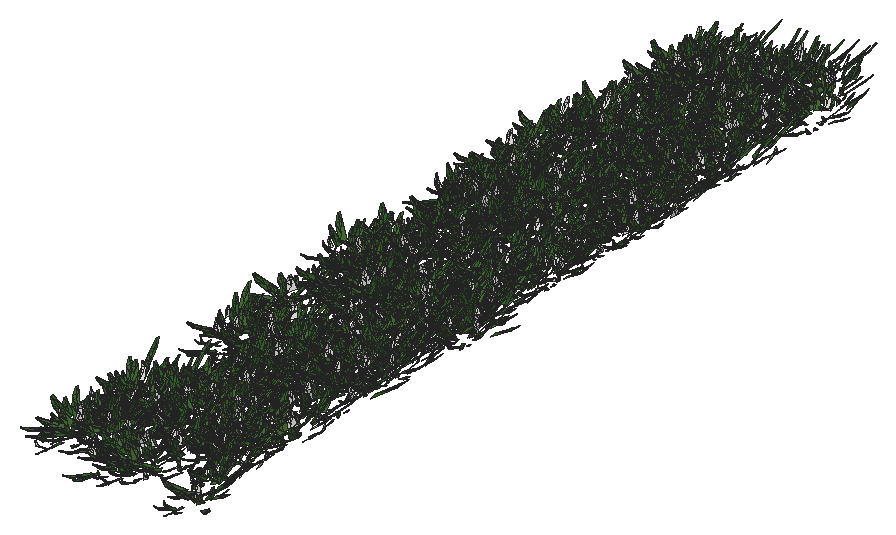
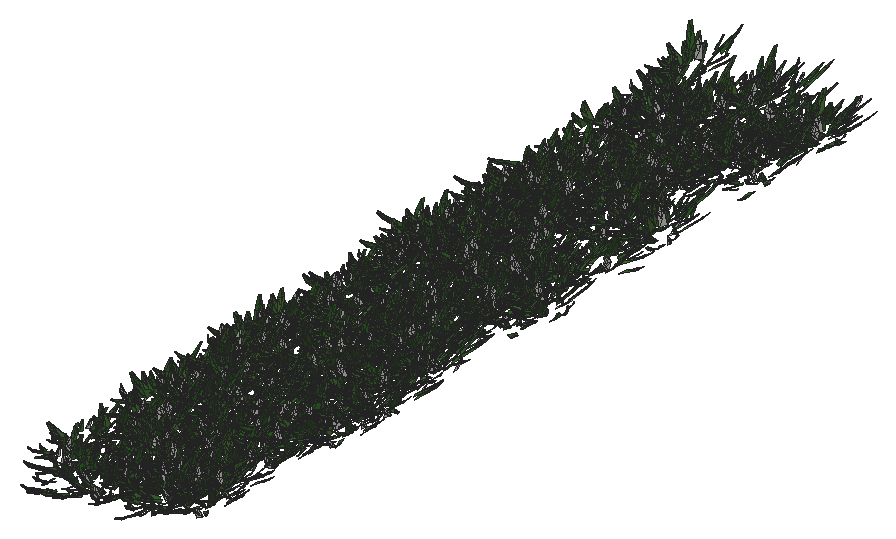
# SketchUp Ruby script. Lengths in inches.
U = 1.inch
M = Sketchup.active_model
def pt(a) = Geom::Point3d.new(a.map { |v| v * U })
def face(e, loops, mat)
  f = e.add_face(loops[0].map { |a| pt(a) })
  loops[1..].each { |l| e.add_face(l.map { |a| pt(a) }).erase! }
  f.material = f.back_material = mat if mat
  f
end
# faces: each face lists its corners as indices into pts; further lists are holes
def faces(e, pts, list, mat = nil) = list.each { |f| face(e, (f[0].is_a?(Array) ? f : [f]).map { |l| l.map { |i| pts[i] } }, mat) }
# xy, xz, yz: faces in a plane at the given z, y or x. An outline is a flat list of corners, or four numbers for a rectangle; further outlines are holes
def ring(l) = l.size == 4 ? [[l[0], l[1]], [l[2], l[1]], [l[2], l[3]], [l[0], l[3]]] : l.each_slice(2).to_a
def flat(e, list, mat, &to3) = list.each { |f| face(e, (f[0].is_a?(Array) ? f : [f]).map { |l| ring(l).map { |u, v| to3.(u, v) } }, mat) }
def xy(e, z, list, mat = nil) = flat(e, list, mat) { |x, y| [x, y, z] }
def xz(e, y, list, mat = nil) = flat(e, list, mat) { |x, z| [x, y, z] }
def yz(e, x, list, mat = nil) = flat(e, list, mat) { |y, z| [x, y, z] }
def lines(e, pts, list) = list.each { |a, b| e.add_line(pt(pts[a]), pt(pts[b])) }
# prism: a flat outline (further loops are holes) pulled along v
def prism(e, loops, v, mat = nil)
  f = face(e, loops, mat); d = Geom::Vector3d.new(v.map { |x| x * U })
  f.pushpull(f.normal.samedirection?(d) ? d.length : -d.length)
end
def box(e, o, s, mat = nil) = prism(e, [[o, [o[0] + s[0], o[1], o[2]], [o[0] + s[0], o[1] + s[1], o[2]], [o[0], o[1] + s[1], o[2]]]], [0, 0, s[2]], mat)
def at(x, y, z, deg = 0) = Geom::Transformation.translation(pt([x, y, z])) * Geom::Transformation.rotation(ORIGIN, Z_AXIS, deg.degrees)
def axes(o, x, y, z) = Geom::Transformation.new([*x, 0, *y, 0, *z, 0, *pt(o).to_a, 1])
def part(name) = M.definitions.add(name)
# library, detail: a bought-in or finely detailed component or shape, given as its bounding box
def library(name, o, s) = part(name).tap { |d| box(d.entities, o, s) }
def detail(e, o, s) = box(e.add_group.entities, o, s)
def put(e, d, t, mat = nil) = e.add_instance(d, t).tap { |i| i.material = mat if mat }
def group(e, t, mat = nil) = e.add_group.tap { |g| g.transformation = t; g.material = mat if mat }.entities
root = M.entities
M.materials.add("Material10").color = [48, 90, 38]
M.materials.add("Material11").color = [68, 110, 48]
M.materials.add("Material12").color = [48, 90, 48]
M.materials.add("Material13").color = [58, 110, 58]
M.materials.add("Material14").color = [58, 90, 38]
M.materials.add("Material15").color = [68, 100, 58]
M.materials.add("Material16").color = [48, 100, 38]
M.materials.add("Material9").color = [68, 110, 58]
c1 = part("grass00")
p = [[-0.6875,0.15,0],[-0.56,0.08,5.52],[-0.04,0.03,2.76],[0.48,-0.02,0],[0.35,-0.02,5.52],[-0.1,-0.14,5.52],
  [-0.12,0.65,8.37],[-0.42,0.65,8.37]]
faces(c1.entities,p,[[0,1,2,3],[3,2,4],[1,5,2],[5,4,2],[1,6,5],[4,5,6],[7,6,1]])
c2 = part("Group16\#1")
put(c2.entities,c1,axes([1.44,-0.61,-0.01],[0.05352,0.12609,0],[-0.10704,0.04543,0.07239],[0.06664,-0.02828,0.11628]),"Material12")
put(c2.entities,c1,axes([0.76,-0.15,-0.01],[0.04676,0.24062,0],[-0.23162,0.04501,0.06642],[0.0652,-0.01267,0.23595]),"Material9")
put(c2.entities,c1,axes([0.79,0.01,-0.01],[-0.00606,0.34651,0],[-0.34381,-0.00602,0.0432],[0.04319,0.00076,0.34386]))
put(c2.entities,c1,axes([1,0.23,-0.01],[-0.07192,0.31144,0],[-0.28722,-0.06632,0.1236],[0.12043,0.02781,0.29478]),"Material11")
put(c2.entities,c1,axes([1.66,0.77,-0.01],[-0.13828,0.29651,0],[-0.21551,-0.1005,0.22471],[0.20365,0.09498,0.23779]),"Material16")
put(c2.entities,c1,axes([0.6875,0.52,-0.01],[-0.18126,0.24051,0],[-0.22746,-0.17142,0.09788],[0.07817,0.05891,0.28481]),"Material11")
put(c2.entities,c1,axes([0.68,0.78,-0.01],[-0.215,0.18688,0],[-0.12385,-0.14248,0.21334],[0.13995,0.16101,0.18878]),"Material9")
put(c2.entities,c1,axes([0.56,1,-0.01],[-0.13756,0.07624,0],[-0.06159,-0.11112,0.0927],[0.04494,0.08108,0.12705]),"Material11")
put(c2.entities,c1,axes([0.2,0.64,-0.01],[-0.23729,0.07254,0],[-0.05711,-0.18681,0.153],[0.04473,0.14632,0.19535]),"Material16")
put(c2.entities,c1,axes([0.0625,0.72,-0.01],[-0.28874,0.02525,0],[-0.02179,-0.24916,0.14647],[0.01276,0.14591,0.25012]),"Material9")
put(c2.entities,c1,axes([-0.08,0.62,-0.01],[-0.34089,-0.04187,0],[0.03255,-0.26504,0.216],[-0.02633,0.21439,0.26703]),"Material16")
put(c2.entities,c1,axes([-0.34,0.98,-0.01],[-0.14314,-0.0493,0],[0.04397,-0.12769,0.06843],[-0.02228,0.0647,0.13505]),"Material16")
put(c2.entities,c1,axes([-0.87,1.45,-0.01],[-0.23488,-0.14114,0],[0.13761,-0.22901,0.06087],[-0.03135,0.05217,0.26717]))
put(c2.entities,c1,axes([-0.72,0.77,-0.01],[-0.14208,-0.13251,0],[0.07209,-0.0773,0.16301],[-0.11118,0.11922,0.1057]),"Material16")
put(c2.entities,c1,axes([-0.62,0.43,-0.01],[-0.14845,-0.21203,0],[0.18654,-0.13061,0.12304],[-0.10079,0.07057,0.22772]),"Material9")
put(c2.entities,c1,axes([-0.68,0.29,-0.01],[-0.13639,-0.32136,0],[0.31723,-0.13464,0.05579],[-0.05136,0.0218,0.34462]),"Material10")
put(c2.entities,c1,axes([-0.64,0.125,-0.01],[-0.0458,-0.23569,0],[0.22124,-0.043,0.08276],[-0.08124,0.01579,0.22538]),"Material13")
put(c2.entities,c1,axes([-1.6,-0.03,-0.01],[0.00576,-0.32897,0],[0.27526,0.00482,0.18018],[-0.18015,-0.00315,0.2753]),"Material11")
put(c2.entities,c1,axes([-1.36,-0.31,-0.01],[0.05718,-0.24765,0],[0.18172,0.04196,0.17267],[-0.16825,-0.03885,0.1865]),"Material16")
put(c2.entities,c1,axes([-1.54,-0.72,-0.01],[0.06537,-0.14017,0],[0.13555,0.06321,0.03939],[-0.0357,-0.01665,0.14956]))
put(c2.entities,c1,axes([-1.19,-0.9,-0.01],[0.09597,-0.12735,0],[0.11214,0.08451,0.07557],[-0.06035,-0.04548,0.14042]),"Material15")
put(c2.entities,c1,axes([-0.47,-0.54,-0.01],[0.11588,-0.10072,0],[0.0618,0.0711,0.12124],[-0.07953,-0.0915,0.0942]))
put(c2.entities,c1,axes([-0.47,-0.84,-0.01],[0.11927,-0.0661,0],[0.06603,0.11913,0.00646],[-0.00313,-0.00565,0.13621]),"Material11")
put(c2.entities,c1,axes([-0.38,-1.24,-0.01],[0.28037,-0.08571,0],[0.0618,0.20215,0.20315],[-0.05939,-0.19428,0.21139]),"Material15")
put(c2.entities,c1,axes([-0.06,-0.66,-0.01],[0.22719,-0.01987,0],[0.01247,0.14255,0.17758],[-0.01547,-0.17691,0.1431]),"Material14")
put(c2.entities,c1,axes([0.11,-0.89,-0.01],[0.14882,0.01828,0],[-0.01058,0.08611,0.12229],[0.01491,-0.12138,0.08676]),"Material12")
put(c2.entities,c1,axes([0.25,-0.72,-0.01],[0.20481,0.07053,0],[-0.06206,0.18022,0.10291],[0.03351,-0.0973,0.1906]),"Material12")
put(c2.entities,c1,axes([0.85,-1.42,-0.01],[0.16481,0.09904,0],[-0.09472,0.15762,0.05616],[0.02893,-0.04814,0.18389]),"Material11")
put(c2.entities,c1,axes([1.01,-1.09,-0.01],[0.21858,0.20385,0],[-0.17495,0.1876,0.15339],[0.10462,-0.11218,0.25652]),"Material16")
put(c2.entities,c1,axes([1.01,-0.71,-0.01],[0.08733,0.12473,0],[-0.06445,0.04512,0.13037],[0.1068,-0.07477,0.07867]),"Material12")
c3 = part("Group15\#1")
put(c3.entities,c2,at(0,0,0))
c4 = part("3darcstudiotree_grass00\#1")
put(c4.entities,c3,at(0,0,0))
put(root,c4,axes([935.18,263.3,12.99],[2.16357,-5.91356,0],[2.30527,4.40706,-0.02296],[0.07841,0.1499,1.8355]))
put(root,c4,axes([915.44,263.39,12.99],[-2.20379,4.7227,0],[-1.94764,-4.7489,-0.04557],[-0.15642,-0.38139,1.96028]))
put(root,c4,axes([909.77,264.4,12.99],[0.55955,7.10793,0],[-3.43066,1.41116,-0.03105],[-0.09608,0.03952,1.50318]))
put(root,c4,axes([890.625,270.69,12.99],[2.4509,-2.72765,0],[1.3443,6.31156,-0.02466],[0.03839,0.18026,1.49812]))
put(root,c4,axes([902.12,270.59,12.99],[3.0266,0.5357,0],[-0.23389,6.90474,-0.0417],[-0.01483,0.43784,1.91485]))
put(root,c4,axes([893.11,269.13,12.99],[-2.69886,4.09648,0],[-1.88583,-6.49197,-0.05111],[-0.09296,-0.32002,1.53759]))
put(root,c4,axes([913.71,270.64,12.99],[-2.55155,1.15726,0],[-0.67109,-7.73133,-0.05548],[-0.03755,-0.43264,1.6451]))
put(root,c4,axes([896.61,273.32,12.99],[2.47649,-1.87564,0],[0.81946,5.65356,-0.03222],[0.0507,0.34977,1.78787]))
put(root,c4,axes([933.94,274.82,12.99],[0.26058,-5.98951,0],[2.59588,0.59011,-0.03727],[0.17952,0.04081,1.73202]))
put(root,c4,axes([922.55,274.69,12.99],[2.18042,5.99333,0],[-2.41636,4.59344,-0.02991],[-0.10428,0.19824,1.95467]))
put(root,c4,axes([915.3,280.95,12.99],[0.84248,-6.06099,0],[3.32927,2.41806,-0.03698],[0.1346,0.09776,1.82987]))
put(root,c4,axes([902.06,280.54,12.99],[2.67334,3.302,0],[-1.601,6.77287,-0.05913],[-0.08489,0.35912,1.39517]))
put(root,c4,axes([925.27,283.74,12.99],[2.64217,1.82812,0],[-0.77048,5.81865,-0.0422],[-0.06297,0.47558,1.87907]))
put(root,c4,axes([894.71,283.2,12.99],[0.30258,5.97975,0],[-2.6892,0.71103,-0.04522],[-0.19467,0.05147,1.60941]))
put(root,c4,axes([927.36,286.8,12.99],[-0.48481,-6.29671,0],[3.40138,-1.36842,-0.05842],[0.24081,-0.09688,1.98292]))
put(root,c4,axes([896.98,287.82,12.99],[0.07451,5.72987,0],[-2.99409,0.20343,-0.05613],[-0.20834,0.01416,1.5259]))
put(root,c4,axes([930.82,288.45,12.99],[-0.59794,6.77866,0],[-3.32974,-1.53473,-0.03197],[-0.12012,-0.05536,1.78572]))
put(root,c4,axes([922.97,288.78,12.99],[-1.61812,4.61984,0],[-2.15897,-3.95126,-0.02462],[-0.09911,-0.18139,1.95656]))
put(root,c4,axes([911.1,290.17,12.99],[0.15448,7.03804,0],[-3.15891,0.3623,-0.03261],[-0.13956,0.01601,1.85888]))
put(root,c4,axes([902.84,291.36,12.99],[-2.83425,-2.19082,0],[1.0252,-6.93022,-0.06149],[0.08094,-0.54714,1.80385]))
put(root,c4,axes([919.43,293.36,12.99],[0.28554,-6.12066,0],[2.58896,0.63109,-0.04937],[0.23664,0.05768,1.72169]))
put(root,c4,axes([890.25,290.95,12.99],[-0.8991,6.69956,0],[-2.48642,-1.74358,-0.03727],[-0.15773,-0.11061,1.57911]))
put(root,c4,axes([906.93,291.31,12.99],[-1.55877,4.2642,0],[-2.16198,-4.12952,-0.03387],[-0.10376,-0.19819,1.54303]))
put(root,c4,axes([900.96,296.68,12.99],[3.19893,-1.82748,0],[0.83009,7.5925,-0.03338],[0.02373,0.21705,1.37691]))
put(root,c4,axes([913.83,298.35,12.99],[3.1357,-0.12665,0],[0.05967,7.7196,-0.02875],[0.00171,0.22117,1.55972]))
put(root,c4,axes([899.2,297.53,12.99],[-1.95357,-4.86449,0],[2.57251,-5.39828,-0.02326],[0.06518,-0.13678,1.82249]))
put(root,c4,axes([917.67,299.18,12.99],[2.85614,0.33498,0],[-0.1772,7.89456,-0.05168],[-0.00943,0.41991,1.68853]))
put(root,c4,axes([906.82,300.59,12.99],[2.46621,-2.49634,0],[1.37227,7.0839,-0.04981],[0.07622,0.39344,1.75709]))
put(root,c4,axes([934.14,299.43,12.99],[-2.54152,0.87828,0],[-0.51281,-7.75401,-0.03474],[-0.01575,-0.23822,1.42794]))
put(root,c4,axes([909.41,310.8,12.99],[2.56753,-3.22377,0],[1.52309,6.33844,-0.02691],[0.05337,0.22209,1.78778]))
put(root,c4,axes([905.07,311.97,12.99],[1.60949,-4.90569,0],[2.62915,4.50723,-0.03529],[0.08496,0.14565,1.35654]))
put(root,c4,axes([919.74,309.36,12.99],[0.30438,6.9191,0],[-2.59362,0.59618,-0.04963],[-0.20426,0.04695,1.47912]))
put(root,c4,axes([926.87,310.41,12.99],[-2.3954,-1.21971,0],[0.57208,-5.87055,-0.02543],[0.0247,-0.25348,1.61262]))
put(root,c4,axes([931.7,317.65,12.99],[3.43264,0.78476,0],[-0.31796,7.26727,-0.02551],[-0.00858,0.19612,1.48132]))
put(root,c4,axes([907.14,315.43,12.99],[-2.59009,-1.18551,0],[0.65428,-7.46927,-0.02406],[0.01587,-0.18113,1.53532]))
put(root,c4,axes([925.55,318.65,12.99],[1.13737,-6.22745,0],[3.14236,2.99884,-0.03949],[0.13997,0.13357,1.7941]))
put(root,c4,axes([913.37,320.24,12.99],[-0.6329,-6.26499,0],[2.41829,-1.27651,-0.0292],[0.1287,-0.06793,1.53984]))
put(root,c4,axes([918.51,319.61,12.99],[-2.31275,-5.6399,0],[2.13118,-4.56649,-0.03051],[0.09167,-0.19643,1.65027]))
put(root,c4,axes([911.11,321.42,12.99],[-2.19766,2.63725,0],[-1.50859,-6.5688,-0.02543],[-0.05069,-0.2207,1.9093]))
put(root,c4,axes([901.46,326.53,12.99],[2.34484,1.67767,0],[-0.78102,5.70392,-0.01935],[-0.03099,0.2263,1.92273]))
put(root,c4,axes([891.36,329.97,12.99],[2.38559,-4.12259,0],[1.77698,5.37296,-0.04167],[0.11572,0.34989,1.86151]))
put(root,c4,axes([925.21,329.9375,12.99],[1.01185,-6.13372,0],[2.94685,2.54013,-0.04892],[0.20515,0.17684,1.93615]))
put(root,c4,axes([921.68,327.36,12.99],[-2.9335,3.57975,0],[-1.49531,-6.40282,-0.03463],[-0.06966,-0.29827,1.86049]))
put(root,c4,axes([895.08,328.11,12.99],[1.03208,6.9747,0],[-2.68336,2.07478,-0.04556],[-0.17093,0.13217,1.53888]))
put(root,c4,axes([905.72,328,12.99],[-2.96853,1.17827,0],[-0.55155,-7.26089,-0.05401],[-0.02759,-0.36324,1.3206]))
put(root,c4,axes([930.96,328.17,12.99],[-2.29387,5.31899,0],[-1.92718,-4.34276,-0.05097],[-0.17689,-0.39861,1.80901]))
put(root,c4,axes([910.85,330.02,12.99],[1.49517,6.0252,0],[-2.13115,2.76336,-0.03898],[-0.2005,0.25998,1.98748]))
put(root,c4,axes([931.32,333.71,12.99],[3.29157,0.19765,0],[-0.0729,6.34378,-0.04419],[-0.00605,0.52622,1.98467]))
put(root,c4,axes([923.25,334.55,12.99],[-1.28092,-6.04021,0],[2.36801,-2.62397,-0.03263],[0.15212,-0.16856,1.87]))
put(root,c4,axes([907.04,334.1,12.99],[0.19188,6.45168,0],[-2.91933,0.45367,-0.02807],[-0.09195,0.01429,1.3177]))
put(root,c4,axes([927.87,336.89,12.99],[-2.64172,-2.94211,0],[1.39255,-6.53349,-0.02869],[0.0547,-0.25663,1.89824]))
put(root,c4,axes([900.78,336.65,12.99],[-2.02503,5.9728,0],[-2.72965,-4.83576,-0.03455],[-0.09116,-0.16149,1.58129]))
put(root,c4,axes([933.45,338.04,12.99],[-0.05703,6.90809,0],[-3.01631,-0.13012,-0.05443],[-0.20637,-0.0089,1.56933]))
put(root,c4,axes([918.78,340.45,12.99],[-2.3608,3.10119,0],[-1.71504,-6.822,-0.04948],[-0.08367,-0.33283,1.60238]))
put(root,c4,axes([930.07,346.93,12.99],[-0.3811,-6.25744,0],[2.92043,-0.92938,-0.04493],[0.21077,-0.06707,1.91565]))
put(root,c4,axes([923.65,346,12.99],[0.6447,7.6773,0],[-3.22798,1.41641,-0.02457],[-0.08545,0.03749,1.59681]))
put(root,c4,axes([913.5625,348.04,12.99],[-2.96012,-3.01306,0],[1.13764,-5.83994,-0.04343],[0.06227,-0.31964,1.35201]))
put(root,c4,axes([892.55,349.5,12.99],[-2.76535,3.02426,0],[-1.42664,-6.81635,-0.05113],[-0.06519,-0.31149,1.33965]))
put(root,c4,axes([926.76,352.58,12.99],[3.25176,-0.12881,0],[0.04504,5.94083,-0.04649],[0.00355,0.46887,1.57333]))
put(root,c4,axes([913.17,353.78,12.99],[1.57024,-6.79737,0],[2.20515,2.66175,-0.03491],[0.14912,0.17999,1.65255]))
put(root,c4,axes([907.45,355.25,12.99],[2.10527,-5.81925,0],[2.05557,3.88578,-0.04304],[0.15955,0.30161,1.76026]))
put(root,c4,axes([917.39,355.44,12.99],[1.08889,6.52286,0],[-2.62742,2.29182,-0.03212],[-0.13469,0.11749,1.73128]))
put(root,c4,axes([929.44,356.81,12.99],[-3.08741,-3.51294,0],[1.5186,-6.97387,-0.0574],[0.07737,-0.3553,1.41402]))
put(root,c4,axes([903.07,358.83,12.99],[-0.6188,5.79492,0],[-2.63413,-1.46975,-0.03757],[-0.12913,-0.07205,1.3158]))
put(root,c4,axes([934.9,362.73,12.99],[3.43357,-1.19868,0],[0.39275,5.87843,-0.02943],[0.01889,0.28266,1.51666]))
put(root,c4,axes([931.8125,363.02,12.99],[1.30473,-5.37131,0],[2.49236,3.16341,-0.03203],[0.12682,0.16096,1.771]))
put(root,c4,axes([927.76,363.33,12.99],[-2.76397,-3.39293,0],[1.26475,-5.38352,-0.0264],[0.0674,-0.28689,1.979]))
put(root,c4,axes([895.02,365.43,12.99],[-0.95226,-7.4517,0],[2.54747,-1.70103,-0.03009],[0.13673,-0.0913,1.72353]))
put(root,c4,axes([915.55,365.98,12.99],[3.45272,-0.50186,0],[0.17621,6.33467,-0.03177],[0.0101,0.36319,1.90853]))
put(root,c4,axes([919.6,363.72,12.99],[-1.19607,6.5176,0],[-2.69105,-2.58045,-0.04701],[-0.19916,-0.19097,1.83905]))
put(root,c4,axes([923.92,366.37,12.99],[0.01926,-5.95035,0],[3.43446,0.05808,-0.04606],[0.17701,0.00299,1.81052]))
put(root,c4,axes([905.76,365.74,12.99],[-3.0211,-1.43467,0],[0.68907,-7.58199,-0.02537],[0.02028,-0.22317,1.82613]))
put(root,c4,axes([903.64,368.53,12.99],[2.27936,-2.55999,0],[1.36933,6.37068,-0.05746],[0.11758,0.54702,1.97658]))
put(root,c4,axes([896.85,367.99,12.99],[-1.45918,-6.19587,0],[2.59618,-3.19483,-0.02018],[0.08577,-0.10555,1.95264]))
put(root,c4,axes([930.375,371.48,12.99],[2.44997,4.15554,0],[-1.70547,5.25389,-0.02502],[-0.07234,0.22284,1.90511]))
put(root,c4,axes([933.6,373.13,12.99],[1.23963,-6.65631,0],[3.16959,3.08438,-0.03539],[0.10455,0.10174,1.51703]))
put(root,c4,axes([899.34,371.82,12.99],[1.13528,6.42669,0],[-2.91025,2.68628,-0.05886],[-0.1698,0.15673,1.33951]))
put(root,c4,axes([915.01,371.28,12.99],[-2.80533,3.90711,0],[-1.57358,-5.90369,-0.05764],[-0.13031,-0.48887,1.8024]))
put(root,c4,axes([890.03,375.21,12.99],[3.16827,-1.89272,0],[0.67082,5.86741,-0.02428],[0.03364,0.2942,1.99391]))
put(root,c4,axes([900.82,372.46,12.99],[-2.12283,6.2438,0],[-2.08381,-3.70193,-0.03149],[-0.0919,-0.16326,1.33797]))
put(root,c4,axes([926.03,377.67,12.99],[-1.87123,-4.95728,0],[2.38433,-4.70279,-0.03179],[0.07424,-0.14642,1.33245]))
put(root,c4,axes([897.51,380.81,12.99],[2.22832,-3.77821,0],[1.70427,5.25211,-0.02804],[0.06628,0.20425,1.55696]))
put(root,c4,axes([925.58,380.51,12.99],[3.35945,-0.32725,0],[0.13167,7.06296,-0.04096],[0.00708,0.37959,1.72127]))
put(root,c4,axes([906.7,381.2,12.99],[-0.51025,-5.78234,0],[3.09016,-1.42483,-0.04603],[0.17303,-0.07978,1.65834]))
put(root,c4,axes([913.13,381.32,12.99],[2.93536,2.92264,0],[-1.15118,6.04135,-0.04191],[-0.05614,0.29462,1.32656]))
put(root,c4,axes([903.12,380.73,12.99],[-2.93795,2.47042,0],[-0.93839,-5.83129,-0.04924],[-0.09044,-0.56198,1.98345]))
put(root,c4,axes([918.61,383.04,12.99],[2.39442,2.70614,0],[-1.19327,5.51686,-0.03066],[-0.06441,0.2978,1.75054]))
put(root,c4,axes([893.09,383.93,12.99],[-1.58543,5.06805,0],[-2.49433,-4.07722,-0.05929],[-0.16235,-0.26538,1.41608]))
put(root,c4,axes([898.27,390.72,12.99],[-2.85671,-2.53106,0],[1.07413,-6.33472,-0.05586],[0.09513,-0.56103,1.92103]))
put(root,c4,axes([931.73,391.05,12.99],[-0.28808,6.00588,0],[-2.73909,-0.6865,-0.02456],[-0.11027,-0.02764,1.70727]))
put(root,c4,axes([923.48,392.41,12.99],[2.10552,4.47167,0],[-1.67922,4.13144,-0.03885],[-0.15269,0.37568,1.95422]))
put(root,c4,axes([913.2,393.76,12.99],[-1.31267,-5.00424,0],[2.30224,-3.15553,-0.04451],[0.1615,-0.22136,1.55797]))
put(root,c4,axes([902.92,396.16,12.99],[-1.52573,-5.90101,0],[2.7304,-3.68878,-0.04139],[0.15126,-0.20436,1.84708]))
put(root,c4,axes([910.55,395.8,12.99],[-2.43393,-1.49333,0],[0.70798,-6.0295,-0.03217],[0.04144,-0.35291,1.86146]))
put(root,c4,axes([933.41,395.26,12.99],[-1.39229,5.31662,0],[-2.61406,-3.57698,-0.03562],[-0.10083,-0.13798,1.37892]))
put(root,c4,axes([901.6875,399.25,12.99],[2.54319,-0.88049,0],[0.50409,7.60787,-0.05863],[0.03157,0.47643,1.66018]))
put(root,c4,axes([932.13,400.13,12.99],[2.46627,-1.94479,0],[0.81477,5.39895,-0.03311],[0.04959,0.32863,1.57439]))
put(root,c4,axes([921.63,401.1,12.99],[2.99394,1.43979,0],[-0.58552,6.36195,-0.04482],[-0.03578,0.38872,1.51278]))
put(root,c4,axes([909.54,402.95,12.99],[1.44359,4.58237,0],[-2.11976,3.48936,-0.02117],[-0.08128,0.1338,1.69559]))
put(root,c4,axes([926.46,404.87,12.99],[3.24081,1.84623,0],[-0.84278,7.73014,-0.03274],[-0.02686,0.24638,1.62193]))
put(root,c4,axes([913.12,404.11,12.99],[-1.81232,-4.45479,0],[1.85093,-3.93462,-0.03633],[0.13307,-0.28288,1.73438]))
put(root,c4,axes([895.43,405.85,12.99],[2.48204,2.31992,0],[-1.16586,6.51758,-0.03911],[-0.05268,0.29452,1.50402]))
put(root,c4,axes([901.16,408.85,12.99],[2.50796,-1.01201,0],[0.56093,7.26362,-0.03701],[0.02885,0.37353,1.98432]))
put(root,c4,axes([922.06,412.6,12.99],[2.35012,-3.0896,0],[1.65108,6.56239,-0.03788],[0.05823,0.23145,1.40078]))
put(root,c4,axes([913.61,410.24,12.99],[1.49184,7.13047,0],[-2.55308,2.79109,-0.02212],[-0.10038,0.10974,1.95299]))
put(root,c4,axes([909.33,410.95,12.99],[-0.11893,6.73443,0],[-3.16025,-0.29163,-0.04298],[-0.18688,-0.01725,1.88799]))
put(root,c4,axes([893.37,412.72,12.99],[0.67663,5.40504,0],[-3.23184,2.11403,-0.02742],[-0.11069,0.07241,1.93645]))
put(root,c4,axes([905.51,412.62,12.99],[-2.87016,2.22055,0],[-0.80799,-5.45703,-0.02484],[-0.04533,-0.30618,1.96802]))
put(root,c4,axes([897.81,414.16,12.99],[1.66242,5.93012,0],[-2.90488,4.2551,-0.02786],[-0.09799,0.14353,1.9768]))
put(root,c4,axes([930.99,414.9,12.99],[-2.37472,-4.8325,0],[1.99955,-5.13427,-0.03256],[0.08529,-0.219,1.62483]))
put(root,c4,axes([897.21,419.75,12.99],[-2.5226,-4.21621,0],[1.48095,-4.62991,-0.03203],[0.1072,-0.33513,1.95145]))
put(root,c4,axes([934.67,418.51,12.99],[-0.39982,6.94288,0],[-2.44789,-0.73658,-0.03263],[-0.14292,-0.04301,1.49628]))
put(root,c4,axes([894.68,420.55,12.99],[-2.87186,-4.44378,0],[1.80504,-6.09539,-0.04034],[0.08321,-0.281,1.62559]))
put(root,c4,axes([909.9,422.13,12.99],[3.35418,0.57967,0],[-0.24666,7.45769,-0.04634],[-0.01548,0.46809,1.98901]))
put(root,c4,axes([913.43,422.65,12.99],[3.04964,1.25386,0],[-0.53495,6.7986,-0.03729],[-0.02558,0.32505,1.60628]))
put(root,c4,axes([932.32,420.55,12.99],[-2.96753,2.96824,0],[-1.23778,-6.46612,-0.02625],[-0.03633,-0.18976,1.46233]))
put(root,c4,axes([919.24,422.77,12.99],[-2.47284,-5.5957,0],[2.42747,-5.60531,-0.03717],[0.10692,-0.24689,1.93537]))
put(root,c4,axes([903.56,424.29,12.99],[1.15052,5.06414,0],[-2.40543,2.85553,-0.04821],[-0.15743,0.18689,1.36797]))
put(root,c4,axes([934.59,430.32,12.99],[0.9483,-5.24975,0],[2.99436,2.8263,-0.04448],[0.17859,0.16856,1.93016]))
put(root,c4,axes([915.16,428.29,12.99],[-1.58054,5.24074,0],[-2.34104,-3.68916,-0.02321],[-0.08331,-0.13128,1.70026]))
put(root,c4,axes([922.45,431.89,12.99],[2.64738,-1.91521,0],[0.78527,5.67185,-0.04021],[0.05245,0.37881,1.5432]))
put(root,c4,axes([902.18,432.54,12.99],[3.43213,-0.14622,0],[0.06184,7.58453,-0.03615],[0.0023,0.28193,1.55355]))
put(root,c4,axes([893.96,433.37,12.99],[1.70158,-4.80585,0],[2.5278,4.67661,-0.0352],[0.11418,0.21125,1.86157]))
put(root,c4,axes([909.44,431.9,12.99],[-2.64592,0.17949,0],[-0.08533,-6.57298,-0.02538],[-0.00332,-0.25609,1.74242]))
put(root,c4,axes([891.29,433.9,12.99],[2.78292,4.03002,0],[-1.59952,5.77152,-0.03414],[-0.06345,0.22894,1.42377]))
put(root,c4,axes([931.05,432.73,12.99],[-2.66078,0.65567,0],[-0.3078,-6.52674,-0.01956],[-0.01051,-0.22283,1.97453]))
put(root,c4,axes([933.93,438.21,12.99],[-2.00829,-5.03961,0],[2.00918,-4.18364,-0.02128],[0.0824,-0.17158,1.95268]))
put(root,c4,axes([930,440.47,12.99],[-2.59745,-3.87681,0],[1.58211,-5.53879,-0.0556],[0.12784,-0.44754,1.66946]))
put(root,c4,axes([892.75,443.2,12.99],[2.17451,-4.76372,0],[2.3546,5.61613,-0.03986],[0.09832,0.23452,1.66404]))
put(root,c4,axes([911.15,441.6,12.99],[1.99628,4.97609,0],[-1.80297,3.77943,-0.03804],[-0.14705,0.30825,1.7602]))
put(root,c4,axes([926.45,441.35,12.99],[-2.1331,4.12656,0],[-2.08295,-5.6261,-0.05904],[-0.1276,-0.34464,1.47981]))
put(root,c4,axes([918.49,441.39,12.99],[-2.32705,5.25953,0],[-1.90468,-4.40339,-0.03762],[-0.1047,-0.24205,1.47105]))
put(root,c4,axes([901.125,446.32,12.99],[0.75387,5.35546,0],[-2.42043,1.78032,-0.0339],[-0.16744,0.12316,1.80984]))
put(root,c4,axes([925.8125,449.52,12.99],[-0.59096,-6.58356,0],[3.16307,-1.48357,-0.03341],[0.13753,-0.0645,1.86102]))
put(root,c4,axes([890.25,449.9,12.99],[2.59641,1.00105,0],[-0.48187,6.53063,-0.03005],[-0.01941,0.26302,1.54341]))
put(root,c4,axes([922.42,448.83,12.99],[-2.425,-4.63515,0],[2.15368,-5.88755,-0.04137],[0.0789,-0.21569,1.36909]))
put(root,c4,axes([906.58,449.36,12.99],[1.7486,5.05737,0],[-2.26791,4.09728,-0.02315],[-0.0753,0.13604,1.64391]))
put(root,c4,axes([911.12,449.73,12.99],[1.6975,4.60254,0],[-1.90052,3.6626,-0.04117],[-0.14328,0.27612,1.55213]))
put(root,c4,axes([918.37,450.5625,12.99],[0.49685,5.57442,0],[-2.72333,1.26831,-0.04728],[-0.19973,0.09302,1.64346]))
put(root,c4,axes([931.73,452.38,12.99],[-2.10871,5.51118,0],[-2.48453,-4.96732,-0.03347],[-0.10651,-0.21295,1.91416]))
put(root,c4,axes([897.39,455.26,12.99],[3.39572,0.94457,0],[-0.404,7.58905,-0.0359],[-0.01777,0.33389,1.88046]))
put(root,c4,axes([927.98,456.83,12.99],[1.28801,5.06742,0],[-2.41842,3.21195,-0.03711],[-0.14164,0.18812,1.69359]))
put(root,c4,axes([931.89,458.34,12.99],[-0.76856,-6.00306,0],[3.23732,-2.16568,-0.04795],[0.15235,-0.10192,1.53186]))
put(root,c4,axes([894.46,458.33,12.99],[-1.98724,-3.69714,0],[2.14753,-6.03154,-0.04334],[0.07873,-0.22111,1.34295]))
put(root,c4,axes([915.6,460.68,12.99],[1.57308,-4.52363,0],[2.67384,4.85851,-0.06111],[0.18186,0.33046,1.78135]))
put(root,c4,axes([921.3,461.06,12.99],[-2.98532,-1.87408,0],[0.70073,-5.83251,-0.02848],[0.03814,-0.31747,1.83531]))
put(root,c4,axes([910.01,461.29,12.99],[0.99921,6.27952,0],[-3.23854,2.69269,-0.0524],[-0.14256,0.11853,1.36852]))
put(root,c4,axes([934.79,466.28,12.99],[-0.22036,-6.62955,0],[3.09668,-0.53782,-0.05563],[0.24494,-0.04254,1.88098]))
put(root,c4,axes([895.02,466.35,12.99],[2.98578,-0.13523,0],[0.05393,6.22203,-0.01855],[0.00191,0.2198,1.93628]))
put(root,c4,axes([903.13,464.89,12.99],[-3.17403,-0.56796,0],[0.25263,-7.37708,-0.05117],[0.01385,-0.40452,1.54048]))
put(root,c4,axes([907.34,467.89,12.99],[-3.31951,-1.20973,0],[0.45245,-6.48729,-0.05098],[0.03404,-0.4881,1.67187]))
put(root,c4,axes([913.19,471.09,12.99],[2.40308,2.32431,0],[-1.0482,5.66272,-0.02719],[-0.0554,0.29927,1.929]))
put(root,c4,axes([923.86,476.03,12.99],[2.68647,-1.74648,0],[0.88065,7.0782,-0.03545],[0.03893,0.31294,1.77295]))
put(root,c4,axes([927.64,474.57,12.99],[-2.9014,-0.31332,0],[0.15888,-7.68751,-0.03065],[0.00617,-0.29841,1.9691]))
put(root,c4,axes([917.89,477.5,12.99],[-0.08541,6.22779,0],[-2.97612,-0.21327,-0.04067],[-0.15268,-0.01094,1.53414]))
put(root,c4,axes([903.66,478.13,12.99],[0.62462,5.44322,0],[-2.97779,1.78551,-0.05161],[-0.17972,0.10776,1.52021]))
put(root,c4,axes([911.41,479.13,12.99],[-3.12826,-2.86332,0],[1.05806,-6.04014,-0.04264],[0.06861,-0.39166,1.69007]))
put(root,c4,axes([895.34,484.6,12.99],[1.19312,-6.85619,0],[3.22269,2.9304,-0.04298],[0.14182,0.12896,1.68954]))
put(root,c4,axes([929.68,485.15,12.99],[-2.9456,0.26169,0],[-0.09898,-5.82135,-0.04521],[-0.00959,-0.56429,1.91035]))
put(root,c4,axes([921.11,487.01,12.99],[-0.29478,-7.66556,0],[2.94783,-0.59233,-0.04765],[0.20585,-0.04136,1.76037]))
put(root,c4,axes([915.6875,489.4,12.99],[2.56912,-2.74144,0],[1.33966,6.56003,-0.02938],[0.04718,0.23103,1.64954]))
put(root,c4,axes([910.68,489.52,12.99],[2.13499,-3.09425,0],[1.42085,5.12263,-0.03299],[0.08626,0.311,1.77748]))
put(root,c4,axes([898.15,487.52,12.99],[-2.76879,4.62726,0],[-1.86292,-5.8246,-0.03994],[-0.10742,-0.33587,1.97331]))
put(root,c4,axes([902.28,488.93,12.99],[-1.87145,5.19563,0],[-2.13857,-4.02502,-0.04557],[-0.17158,-0.32292,1.85346]))
put(root,c4,axes([897.08,494.67,12.99],[1.65064,-5.15835,0],[2.07206,3.46456,-0.02877],[0.09832,0.16439,1.49076]))
put(root,c4,axes([905.16,494.99,12.99],[3.09418,1.26168,0],[-0.46203,5.9207,-0.04495],[-0.04328,0.55456,1.97854]))
put(root,c4,axes([935.03,494.61,12.99],[-0.71957,5.72426,0],[-3.33127,-2.1881,-0.06106],[-0.18182,-0.11942,1.47293]))
put(root,c4,axes([910.58,495.75,12.99],[1.42848,4.62835,0],[-2.00366,3.23129,-0.03223],[-0.10781,0.17386,1.37708]))
put(root,c4,axes([900.95,497.33,12.99],[-1.8428,-4.07047,0],[2.10493,-4.97939,-0.03177],[0.09641,-0.22805,1.8145]))
put(root,c4,axes([894.22,498.37,12.99],[2.82593,1.90367,0],[-0.69398,5.38296,-0.026],[-0.03482,0.2701,1.59572]))
put(root,c4,axes([913.56,498.45,12.99],[0.34158,6.08375,0],[-2.98204,0.87487,-0.0516],[-0.24787,0.07272,1.99718]))
put(root,c4,axes([903.4,503.36,12.99],[-2.35584,-2.06993,0],[1.07753,-6.40807,-0.04802],[0.06473,-0.38497,1.54794]))
put(root,c4,axes([913.53,504.68,12.99],[-2.02426,-3.20223,0],[1.52417,-5.03446,-0.03348],[0.09718,-0.32101,1.87437]))
put(root,c4,axes([923.87,505.92,12.99],[-1.49465,-6.74053,0],[2.23858,-2.59372,-0.03791],[0.18527,-0.21466,1.88609]))
put(root,c4,axes([930.64,504.57,12.99],[-2.33353,3.55843,0],[-1.43711,-4.92434,-0.03251],[-0.09102,-0.31189,1.79208]))
put(root,c4,axes([919.24,507.21,12.99],[2.13097,2.75892,0],[-1.30336,5.26026,-0.02459],[-0.06374,0.25725,1.90817]))
